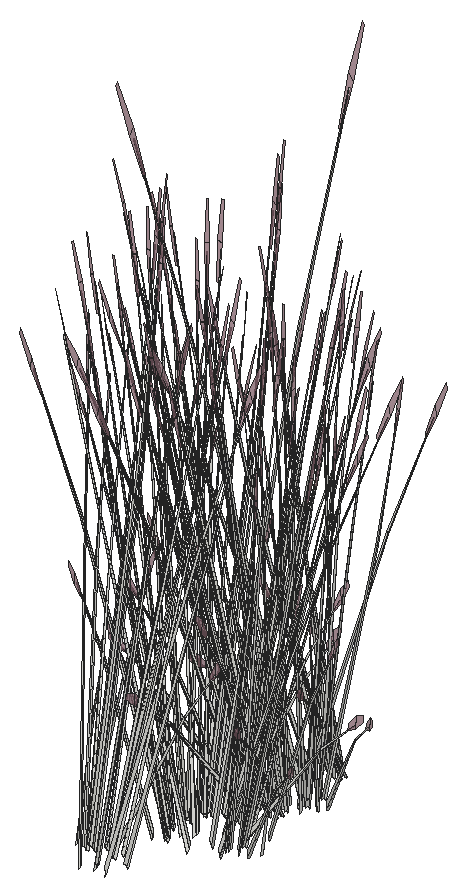
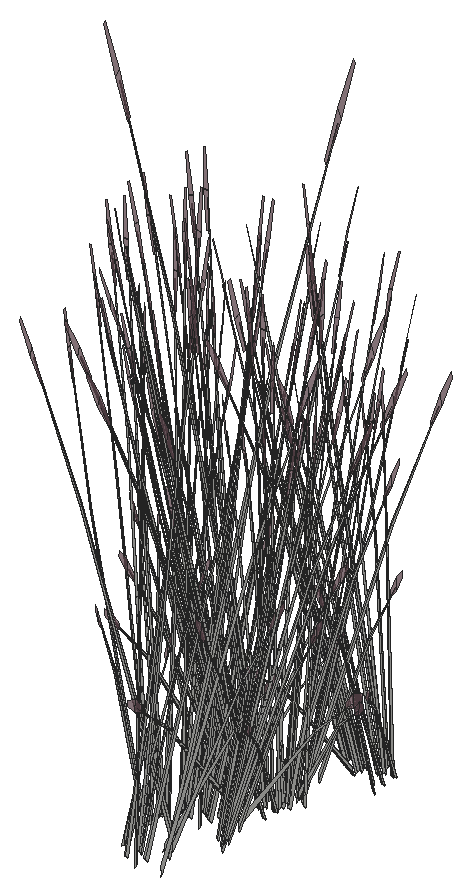
# SketchUp Ruby script. Lengths in inches.
U = 1.inch
M = Sketchup.active_model
def pt(a) = Geom::Point3d.new(a.map { |v| v * U })
def face(e, loops, mat)
  f = e.add_face(loops[0].map { |a| pt(a) })
  loops[1..].each { |l| e.add_face(l.map { |a| pt(a) }).erase! }
  f.material = f.back_material = mat if mat
  f
end
# faces: each face lists its corners as indices into pts; further lists are holes
def faces(e, pts, list, mat = nil) = list.each { |f| face(e, (f[0].is_a?(Array) ? f : [f]).map { |l| l.map { |i| pts[i] } }, mat) }
# xy, xz, yz: faces in a plane at the given z, y or x. An outline is a flat list of corners, or four numbers for a rectangle; further outlines are holes
def ring(l) = l.size == 4 ? [[l[0], l[1]], [l[2], l[1]], [l[2], l[3]], [l[0], l[3]]] : l.each_slice(2).to_a
def flat(e, list, mat, &to3) = list.each { |f| face(e, (f[0].is_a?(Array) ? f : [f]).map { |l| ring(l).map { |u, v| to3.(u, v) } }, mat) }
def xy(e, z, list, mat = nil) = flat(e, list, mat) { |x, y| [x, y, z] }
def xz(e, y, list, mat = nil) = flat(e, list, mat) { |x, z| [x, y, z] }
def yz(e, x, list, mat = nil) = flat(e, list, mat) { |y, z| [x, y, z] }
def lines(e, pts, list) = list.each { |a, b| e.add_line(pt(pts[a]), pt(pts[b])) }
# prism: a flat outline (further loops are holes) pulled along v
def prism(e, loops, v, mat = nil)
  f = face(e, loops, mat); d = Geom::Vector3d.new(v.map { |x| x * U })
  f.pushpull(f.normal.samedirection?(d) ? d.length : -d.length)
end
def box(e, o, s, mat = nil) = prism(e, [[o, [o[0] + s[0], o[1], o[2]], [o[0] + s[0], o[1] + s[1], o[2]], [o[0], o[1] + s[1], o[2]]]], [0, 0, s[2]], mat)
def at(x, y, z, deg = 0) = Geom::Transformation.translation(pt([x, y, z])) * Geom::Transformation.rotation(ORIGIN, Z_AXIS, deg.degrees)
def axes(o, x, y, z) = Geom::Transformation.new([*x, 0, *y, 0, *z, 0, *pt(o).to_a, 1])
def part(name) = M.definitions.add(name)
# library, detail: a bought-in or finely detailed component or shape, given as its bounding box
def library(name, o, s) = part(name).tap { |d| box(d.entities, o, s) }
def detail(e, o, s) = box(e.add_group.entities, o, s)
def put(e, d, t, mat = nil) = e.add_instance(d, t).tap { |i| i.material = mat if mat }
def group(e, t, mat = nil) = e.add_group.tap { |g| g.transformation = t; g.material = mat if mat }.entities
root = M.entities
M.materials.add("LightPink_Translucent").color = [144, 107, 117]
M.materials["LightPink_Translucent"].alpha = 0.75
c1 = part("blade")
p = [[2.15,0.21,22],[0,0.17,0],[0.09,0.45,0],[2.18,0.31,22],[2.29,0.31,22],[0.38,0.45,0],
  [2.48,0.24,33],[2.49,0.24,33],[2.48,0.22,33]]
faces(c1.entities,p,[[0,1,2,3],[4,5,2,3],[6,3,4,7],[8,0,3,6]])
c2 = part("seeds")
p = [[0.3,-0.1,1.38],[-0.01,-0.03,1.59],[-0.01,-0.03,0.03],[0.14,-0.07,-0.07],[0.29,-0.03,3],[0.15,0.01,3.11]]
faces(c2.entities,p,[[0,1,2,3],[1,0,4,5]],"LightPink_Translucent")
c3 = part("blade with seeds")
put(c3.entities,c1,at(0,0,0))
put(c3.entities,c2,axes([2.4,0.25,30.99],[1.5799,-0.05474,1.17369],[-0.12525,1.92788,0.29478],[-0.07173,-0.02425,1.56792]))
put(root,c3,axes([425.38,418,154],[-0.33677,-0.02198,0.05432],[0.00923,-0.33185,0.42765],[-0.03524,0.12712,0.65209]))
put(root,c3,axes([427.53,418.12,153.95],[0.40438,-0.11212,-0.43168],[0.07074,0.4246,-0.33437],[0.10862,0.12168,0.82598]))
put(root,c3,axes([427.33,418.47,154],[-0.18625,0.29962,0.05432],[-0.26523,-0.17444,0.42765],[0.08575,0.09606,0.65209]))
put(root,c3,axes([431.01,421.96,154],[0.28133,0.19836,0.05432],[-0.16379,0.28248,0.42765],[0.0902,-0.09132,0.65209]))
put(root,c3,axes([430.93,421.87,154],[0.10163,0.43409,0.40553],[-0.39868,0.07534,0.33437],[0.1175,-0.10209,0.83914]))
put(root,c3,axes([432.01,422.4,153.98],[0.05687,-0.07184,1.47793],[-0.07279,-0.44069,-0.23373],[0.14268,-0.08356,0.11853]))
put(root,c3,axes([425.4,417.21,153.27],[0.0763,-0.16212,1.44779],[0.3201,0.3355,0.11706],[-0.1444,0.2091,0.61892]))
put(root,c3,axes([427.2,420.68,153.98],[0.03038,0.04707,1.49853],[-0.14646,0.42312,-0.1416],[-0.14833,0.00306,0.26519]))
put(root,c3,axes([426.3,418.51,154],[-0.30197,0.1603,0.05432],[-0.1478,-0.29231,0.42765],[0.02916,0.12885,0.65209]))
put(root,c3,axes([425.49,418.125,153.82],[-0.27728,0.24833,-0.29918],[-0.26248,-0.28355,0.38624],[-0.03994,0.14407,0.73904]))
put(root,c3,axes([424.53,418.05,153.98],[-0.01019,0.09334,1.47793],[0.28908,0.3247,-0.23373],[-0.07568,0.15355,0.11853]))
put(root,c3,axes([425.46,417.84,154.56],[0.45039,0.02337,-0.11403],[-0.01231,0.44247,-0.63292],[-0.03129,0.17041,0.9617]))
put(root,c3,axes([426.29,418.34,154.25],[0.40102,-0.2196,-0.10273],[0.19707,0.38974,-0.57019],[0.05291,0.16424,0.8664]))
put(root,c3,axes([427.625,421.55,153.95],[-0.29757,0.31243,-0.43168],[-0.2606,-0.33005,-0.33437],[-0.15119,-0.04754,0.82598]))
put(root,c3,axes([427.78,421.23,154.25],[-0.02194,0.47967,-0.10273],[-0.41546,-0.01311,-0.57019],[-0.16001,-0.03332,0.8664]))
put(root,c3,axes([430.89,423.07,154.25],[-0.20619,-0.42709,-0.10273],[0.36595,-0.20988,-0.57019],[0.15422,-0.05635,0.8664]))
put(root,c3,axes([430.87,422.7,153.95],[0.11102,-0.42903,-0.43168],[0.38064,0.14706,-0.33437],[0.15325,-0.03934,0.82598]))
put(root,c3,axes([425.76,418.01,154.23],[0.29336,0.31691,-0.47917],[-0.3099,0.27755,-0.37115],[-0.04464,0.16102,0.91684]))
put(root,c3,axes([427.25,421.89,153.27],[0.16998,-0.01068,1.44779],[-0.11276,0.46299,0.11706],[-0.24224,-0.02864,0.61892]))
put(root,c3,axes([426.63,418.32,153.95],[0.40284,0.11824,-0.43168],[-0.13808,0.40538,-0.33437],[0.03694,0.16321,0.82598]))
put(root,c3,axes([426.86,417.48,153.27],[-0.09368,-0.15143,1.44779],[0.43286,-0.12749,0.11706],[0.09783,0.23774,0.61892]))
put(root,c3,axes([426.45,418.57,153.82],[-0.12355,0.36271,-0.29918],[-0.36044,-0.10579,0.38624],[0.03305,0.14603,0.73904]))
put(root,c3,axes([425.67,417.86,154.51],[-0.01066,0.43628,-0.66621],[-0.44902,-0.0293,0.0804],[-0.04739,0.18483,0.94242]))
put(root,c3,axes([424.5,419.01,153.98],[0.04649,-0.02848,1.49853],[0.38427,0.18941,-0.1416],[-0.00903,0.15771,0.26519]))
put(root,c3,axes([426.1,417.55,153.27],[-0.01003,-0.18103,1.44779],[0.43473,0.12009,0.11706],[-0.02689,0.25798,0.61892]))
put(root,c3,axes([427.18,422.24,154],[0.11578,-0.43006,0.40553],[0.38064,0.14706,0.33437],[-0.14969,0.02584,0.83914]))
put(root,c3,axes([427.15,422.12,154],[-0.15051,-0.3216,0.05432],[0.27447,-0.15741,0.42765],[-0.12099,0.03106,0.65209]))
put(root,c3,axes([426.49,418.24,154.21],[0.19559,0.38351,-0.60019],[-0.40262,0.21373,0.07243],[0.04574,0.1853,0.84903]))
put(root,c3,axes([426.19,419.21,153.98],[0.05195,0.07595,1.47793],[0.41921,0.02984,-0.23373],[0.04216,0.1675,0.11853]))
put(root,c3,axes([431.1,422.9,153.82],[0.34057,0.13158,-0.29918],[-0.09933,0.38387,0.38624],[0.13712,-0.0352,0.73904]))
put(root,c3,axes([427.1,422.28,153.82],[-0.34057,-0.13158,-0.29918],[0.09933,-0.38387,0.38624],[-0.13712,0.0352,0.73904]))
put(root,c3,axes([428.2,426.78,153.27],[0.09368,0.15143,1.44779],[-0.43286,0.12749,0.11706],[-0.09783,-0.23774,0.61892]))
put(root,c3,axes([428.91,425.78,153.98],[-0.06268,-0.06613,1.47793],[-0.4183,0.04193,-0.23373],[-0.06676,-0.15817,0.11853]))
put(root,c3,axes([425.52,418.48,152.84],[0.009,-0.24349,1.30391],[0.40497,0.12861,0.18019],[-0.03509,0.2595,0.61571]))
put(root,c3,axes([430.18,422.42,153.27],[-0.16998,0.01068,1.44779],[0.11276,-0.46299,0.11706],[0.24224,0.02864,0.61892]))
put(root,c3,axes([431.05,423.06,154],[0.15051,0.3216,0.05432],[-0.27447,0.15741,0.42765],[0.12099,-0.03106,0.65209]))
put(root,c3,axes([431.03,422.94,154],[-0.11578,0.43006,0.40553],[-0.38064,-0.14706,0.33437],[0.14969,-0.02584,0.83914]))
put(root,c3,axes([428.14,422.22,152.82],[0.11649,-0.06823,1.49584],[0.04017,0.47639,0.11706],[-0.25231,0.06321,0.53462]))
put(root,c3,axes([430.79,426.59,153.98],[-0.00396,-0.09387,1.47793],[-0.33411,-0.2713,-0.23373],[0.05166,-0.16446,0.11853]))
put(root,c3,axes([429.39,426.57,153.82],[0.12355,-0.36271,-0.29918],[0.36044,0.10579,0.38624],[-0.03305,-0.14603,0.73904]))
put(root,c3,axes([429.66,427.05,153.27],[-0.0763,0.16212,1.44779],[-0.3201,-0.3355,0.11706],[0.1444,-0.2091,0.61892]))
put(root,c3,axes([430.7,426.25,153.98],[-0.04162,0.03603,1.49853],[-0.40776,-0.12155,-0.1416],[-0.01476,-0.15722,0.26519]))
put(root,c3,axes([429.21,426.82,153.95],[-0.40284,-0.11824,-0.43168],[0.13808,-0.40538,-0.33437],[-0.03694,-0.16321,0.82598]))
put(root,c3,axes([431.71,424.34,153.98],[-0.03706,-0.04129,1.49853],[0.08106,-0.44261,-0.1416],[0.14596,-0.02828,0.26519]))
put(root,c3,axes([430.08,427.125,153.95],[-0.29336,-0.31691,-0.43168],[0.3099,-0.27755,-0.33437],[0.04464,-0.16102,0.82598]))
put(root,c3,axes([426.89,422.54,153.98],[-0.06692,0.06124,1.47793],[0.00569,0.44742,-0.23373],[-0.15339,0.05818,0.11853]))
put(root,c3,axes([427.34,422.48,153.95],[-0.11102,0.42903,-0.43168],[-0.38064,-0.14706,-0.33437],[-0.15325,0.03934,0.82598]))
put(root,c3,axes([428.49,425.5625,153.98],[-0.00765,0.05653,1.49853],[-0.37706,0.20517,-0.1416],[-0.11096,-0.10488,0.26519]))
put(root,c3,axes([427.32,422.11,154.25],[0.20619,0.42709,-0.10273],[-0.36595,0.20988,-0.57019],[-0.15422,0.05635,0.8664]))
put(root,c3,axes([431.39,423.97,153.32],[-0.07843,-0.39649,-0.0295],[0.37072,-0.09115,-0.13375],[0.07742,0.02514,0.44114]))
put(root,c3,axes([430.43,423.95,154.25],[0.02194,-0.47967,-0.10273],[0.41546,0.01311,-0.57019],[0.16001,0.03332,0.8664]))
put(root,c3,axes([429.43,426.65,154],[0.4038,0.12331,0.40553],[-0.13808,0.40538,0.33437],[-0.02427,-0.15942,0.83914]))
put(root,c3,axes([429.55,426.8,154.25],[-0.40102,0.2196,-0.10273],[-0.19707,-0.38974,-0.57019],[-0.05291,-0.16424,0.8664]))
put(root,c3,axes([430.38,427.29,154.25],[-0.45039,-0.02337,-0.10273],[0.01231,-0.44247,-0.57019],[0.03129,-0.17041,0.8664]))
put(root,c3,axes([430.35,427.01,153.82],[0.27728,-0.24833,-0.29918],[0.26248,0.28355,0.38624],[0.03994,-0.14407,0.73904]))
put(root,c3,axes([429.54,426.62,154],[0.30197,-0.1603,0.05432],[0.1478,0.29231,0.42765],[-0.02916,-0.12885,0.65209]))
put(root,c3,axes([428.35,426.7,153.82],[-0.06329,-0.37991,-0.29918],[0.36182,-0.10032,0.38624],[-0.09718,-0.10887,0.73904]))
put(root,c3,axes([430.79,423.67,153.98],[0.08791,-0.00798,1.47793],[0.24113,-0.36643,-0.23373],[0.15637,0.04837,0.11853]))
put(root,c3,axes([427.27,423.31,154],[-0.10163,-0.43409,0.40553],[0.39868,-0.07534,0.33437],[-0.1175,0.10209,0.83914]))
put(root,c3,axes([428.51,426.67,154],[0.18625,-0.29962,0.05432],[0.26523,0.17444,0.42765],[-0.08575,-0.09606,0.65209]))
put(root,c3,axes([427.19,423.22,154],[-0.28133,-0.19836,0.05432],[0.16379,-0.28248,0.42765],[-0.0902,0.09132,0.65209]))
put(root,c3,axes([427.32,422.7,153.27],[0.14219,-0.09977,1.44779],[0.11971,0.461,0.11706],[-0.22323,0.10419,0.61892]))
put(root,c3,axes([427.57,427.25,153.27],[0.15222,0.08126,1.44779],[-0.31502,0.34091,0.11706],[-0.19634,-0.15379,0.61892]))
put(root,c3,axes([428.31,427.02,153.95],[-0.40438,0.11212,-0.43168],[-0.07074,-0.4246,-0.33437],[-0.10862,-0.12168,0.82598]))
put(root,c3,axes([430.35,427.1,154],[0.29182,0.32181,0.40553],[-0.3099,0.27755,0.33437],[0.05383,-0.15098,0.83914]))
put(root,c3,axes([428.59,426.64,154.59],[-0.2735,0.45217,-0.11506],[-0.39608,-0.2605,-0.63862],[-0.13768,-0.12775,0.97037]))
put(root,c3,axes([430.46,427.14,154],[0.33677,0.02198,0.05432],[-0.00923,0.33185,0.42765],[0.03524,-0.12712,0.65209]))
put(root,c3,axes([426.14,422.99,153.98],[0.0523,0.01265,1.49853],[0.16179,0.41674,-0.1416],[-0.10706,0.10938,0.26519]))
put(root,c3,axes([430.6875,427.86,153.95],[-0.10528,-0.43067,-0.43168],[0.39868,-0.07534,-0.33437],[0.11425,-0.11568,0.82598]))
put(root,c3,axes([430.69,423.92,153.82],[0.23317,0.29531,-0.29918],[-0.26625,0.27955,0.38624],[0.13527,0.04253,0.73904]))
put(root,c3,axes([430.57,424.03,154],[-0.02064,0.35866,0.05432],[-0.3116,-0.00983,0.42765],[0.11936,0.03753,0.65209]))
put(root,c3,axes([427.23,423.39,153.82],[-0.35672,0.06741,-0.29918],[-0.09419,-0.38534,0.38624],[-0.10222,0.1035,0.73904]))
put(root,c3,axes([430.6,423.92,154],[-0.30217,0.31079,0.40553],[-0.2606,-0.33005,0.33437],[0.14177,0.05733,0.83914]))
put(root,c3,axes([427.54,426.51,153.98],[-0.08817,-0.00333,1.47793],[-0.28072,0.33293,-0.23373],[-0.14978,-0.06803,0.11853]))
put(root,c3,axes([430.875,428.16,154.25],[-0.37908,-0.26007,-0.10273],[0.21839,-0.37663,-0.57019],[0.1071,-0.13092,0.8664]))
put(root,c3,axes([429.31,429.58,152.81],[0.35414,0.19019,1.27785],[-0.34693,0.40974,0.50532],[-0.1554,-0.24285,1.07126]))
put(root,c3,axes([431.81,428.05,153.98],[-0.05353,-0.00358,1.49853],[-0.22227,-0.38383,-0.1416],[0.08926,-0.1262,0.26519]))
put(root,c3,axes([429.86,423.16,153.27],[-0.15222,-0.08126,1.44779],[0.31502,-0.34091,0.11706],[0.19634,0.15379,0.61892]))
put(root,c3,axes([429.88,422.09,153.78],[-0.35411,-0.24507,1.16821],[0.37391,-0.38156,0.50405],[0.11425,0.22994,1.12919]))
put(root,c3,axes([427.33,423.13,154.25],[0.37908,0.26007,-0.10273],[-0.21839,0.37663,-0.57019],[-0.1071,0.13092,0.8664]))
put(root,c3,axes([429.61,424.48,154.25],[0.2442,-0.40372,-0.10273],[0.35364,0.23259,-0.57019],[0.12293,0.11406,0.8664]))
put(root,c3,axes([430.98,427.9,153.82],[0.35672,-0.06741,-0.29918],[0.09419,0.38534,0.38624],[0.10222,-0.1035,0.73904]))
put(root,c3,axes([427.63,427.26,154],[0.02064,-0.35866,0.05432],[0.3116,0.00983,0.42765],[-0.11936,-0.03753,0.65209]))
put(root,c3,axes([427.84,423.01,153.27],[0.10236,-0.14492,1.44779],[0.25844,0.39118,0.11706],[-0.17726,0.17814,0.61892]))
put(root,c3,axes([427.51,427.37,153.82],[-0.23317,-0.29531,-0.29918],[0.26625,-0.27955,0.38624],[-0.13527,-0.04253,0.73904]))
put(root,c3,axes([427.52,423.4375,153.95],[0.10528,0.43067,-0.43168],[-0.39868,0.07534,-0.33437],[-0.11425,0.11568,0.82598]))
put(root,c3,axes([429.29,424.8125,153.98],[0.00121,-0.0571,1.49853],[0.35119,-0.25193,-0.1416],[0.12199,0.08992,0.26519]))
put(root,c3,axes([427.75,424.16,154],[-0.33677,-0.02198,0.05432],[0.00923,-0.33185,0.42765],[-0.03524,0.12712,0.65209]))
put(root,c3,axes([427.85,424.1875,154],[-0.29182,-0.32181,0.40553],[0.3099,-0.27755,0.33437],[-0.05383,0.15098,0.83914]))
put(root,c3,axes([429.9,424.28,153.95],[0.40438,-0.11212,-0.43168],[0.07074,0.4246,-0.33437],[0.10862,0.12168,0.82598]))
put(root,c3,axes([431.01,428.07,154],[0.28133,0.19836,0.05432],[-0.16379,0.28248,0.42765],[0.0902,-0.09132,0.65209]))
put(root,c3,axes([429.7,424.625,154],[-0.18625,0.29962,0.05432],[-0.26523,-0.17444,0.42765],[0.08575,0.09606,0.65209]))
put(root,c3,axes([430.93,427.98,154],[0.10163,0.43409,0.40553],[-0.39868,0.07534,0.33437],[0.1175,-0.10209,0.83914]))
put(root,c3,axes([432.01,428.51,153.98],[0.05687,-0.07184,1.47793],[-0.07279,-0.44069,-0.23373],[0.14268,-0.08356,0.11853]))
put(root,c3,axes([429.78,424.54,154],[-0.4076,0.10824,0.40553],[-0.07074,-0.4246,0.33437],[0.09586,0.12514,0.83914]))
put(root,c3,axes([427.77,423.37,153.27],[0.0763,-0.16212,1.44779],[0.3201,0.3355,0.11706],[-0.1444,0.2091,0.61892]))
put(root,c3,axes([427.2,426.79,153.98],[0.03038,0.04707,1.49853],[-0.14646,0.42312,-0.1416],[-0.14833,0.00306,0.26519]))
put(root,c3,axes([428.66,424.67,154],[-0.30197,0.1603,0.05432],[-0.1478,-0.29231,0.42765],[0.02916,0.12885,0.65209]))
put(root,c3,axes([427.625,427.66,153.95],[-0.29757,0.31243,-0.43168],[-0.2606,-0.33005,-0.33437],[-0.15119,-0.04754,0.82598]))
put(root,c3,axes([427.85,424.28,153.82],[-0.27728,0.24833,-0.29918],[-0.26248,-0.28355,0.38624],[-0.03994,0.14407,0.73904]))
put(root,c3,axes([426.9,424.21,153.98],[-0.01019,0.09334,1.47793],[0.28908,0.3247,-0.23373],[-0.07568,0.15355,0.11853]))
put(root,c3,axes([427.82,424,154.56],[0.45039,0.02337,-0.11403],[-0.01231,0.44247,-0.63292],[-0.03129,0.17041,0.9617]))
put(root,c3,axes([428.66,424.49,154.25],[0.40102,-0.2196,-0.10273],[0.19707,0.38974,-0.57019],[0.05291,0.16424,0.8664]))
put(root,c3,axes([427.78,427.34,154.25],[-0.02194,0.47967,-0.10273],[-0.41546,-0.01311,-0.57019],[-0.16001,-0.03332,0.8664]))
put(root,c3,axes([430.89,429.18,154.25],[-0.20619,-0.42709,-0.10273],[0.36595,-0.20988,-0.57019],[0.15422,-0.05635,0.8664]))
put(root,c3,axes([430.87,428.8125,153.95],[0.11102,-0.42903,-0.43168],[0.38064,0.14706,-0.33437],[0.15325,-0.03934,0.82598]))
put(root,c3,axes([427.25,428,153.27],[0.16998,-0.01068,1.44779],[-0.11276,0.46299,0.11706],[-0.24224,-0.02864,0.61892]))
put(root,c3,axes([428.13,424.17,154.23],[0.29336,0.31691,-0.47917],[-0.3099,0.27755,-0.37115],[-0.04464,0.16102,0.91684]))
put(root,c3,axes([428.2,431.7,153.27],[0.09368,0.15143,1.44779],[-0.43286,0.12749,0.11706],[-0.09783,-0.23774,0.61892]))
put(root,c3,axes([429,424.47,153.95],[0.40284,0.11824,-0.43168],[-0.13808,0.40538,-0.33437],[0.03694,0.16321,0.82598]))
put(root,c3,axes([429.23,423.64,153.27],[-0.09368,-0.15143,1.44779],[0.43286,-0.12749,0.11706],[0.09783,0.23774,0.61892]))
put(root,c3,axes([428.91,430.69,153.98],[-0.06268,-0.06613,1.47793],[-0.4183,0.04193,-0.23373],[-0.06676,-0.15817,0.11853]))
put(root,c3,axes([428.82,424.72,153.82],[-0.12355,0.36271,-0.29918],[-0.36044,-0.10579,0.38624],[0.03305,0.14603,0.73904]))
put(root,c3,axes([428.04,424.02,154.51],[-0.01066,0.43628,-0.66621],[-0.44902,-0.0293,0.0804],[-0.04739,0.18483,0.94242]))
put(root,c3,axes([426.87,425.17,153.98],[0.04649,-0.02848,1.49853],[0.38427,0.18941,-0.1416],[-0.00903,0.15771,0.26519]))
put(root,c3,axes([428.46,423.71,153.27],[-0.01003,-0.18103,1.44779],[0.43473,0.12009,0.11706],[-0.02689,0.25798,0.61892]))
put(root,c3,axes([427.18,428.35,154],[0.11578,-0.43006,0.40553],[0.38064,0.14706,0.33437],[-0.14969,0.02584,0.83914]))
put(root,c3,axes([427.15,428.23,154],[-0.15051,-0.3216,0.05432],[0.27447,-0.15741,0.42765],[-0.12099,0.03106,0.65209]))
put(root,c3,axes([430.79,431.5,153.98],[-0.00396,-0.09387,1.47793],[-0.33411,-0.2713,-0.23373],[0.05166,-0.16446,0.11853]))
put(root,c3,axes([429.39,431.48,153.82],[0.12355,-0.36271,-0.29918],[0.36044,0.10579,0.38624],[-0.03305,-0.14603,0.73904]))
put(root,c3,axes([429.66,431.96,153.27],[-0.0763,0.16212,1.44779],[-0.3201,-0.3355,0.11706],[0.1444,-0.2091,0.61892]))
put(root,c3,axes([430.7,431.17,153.98],[-0.04162,0.03603,1.49853],[-0.40776,-0.12155,-0.1416],[-0.01476,-0.15722,0.26519]))
put(root,c3,axes([428.5625,425.36,153.98],[0.05195,0.07595,1.47793],[0.41921,0.02984,-0.23373],[0.04216,0.1675,0.11853]))
put(root,c3,axes([429.21,431.73,153.95],[-0.40284,-0.11824,-0.43168],[0.13808,-0.40538,-0.33437],[-0.03694,-0.16321,0.82598]))
put(root,c3,axes([430.08,432.04,153.95],[-0.29336,-0.31691,-0.43168],[0.3099,-0.27755,-0.33437],[0.04464,-0.16102,0.82598]))
put(root,c3,axes([431.1,429.01,153.82],[0.34057,0.13158,-0.29918],[-0.09933,0.38387,0.38624],[0.13712,-0.0352,0.73904]))
put(root,c3,axes([428.49,430.48,153.98],[-0.00765,0.05653,1.49853],[-0.37706,0.20517,-0.1416],[-0.11096,-0.10488,0.26519]))
put(root,c3,axes([427.1,428.4,153.82],[-0.34057,-0.13158,-0.29918],[0.09933,-0.38387,0.38624],[-0.13712,0.0352,0.73904]))
put(root,c3,axes([429.43,431.57,154],[0.4038,0.12331,0.40553],[-0.13808,0.40538,0.33437],[-0.02427,-0.15942,0.83914]))
put(root,c3,axes([430.18,428.53,153.27],[-0.16998,0.01068,1.44779],[0.11276,-0.46299,0.11706],[0.24224,0.02864,0.61892]))
